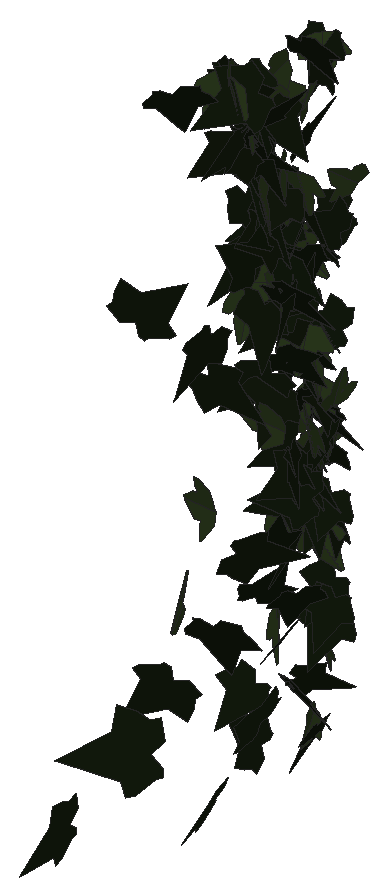
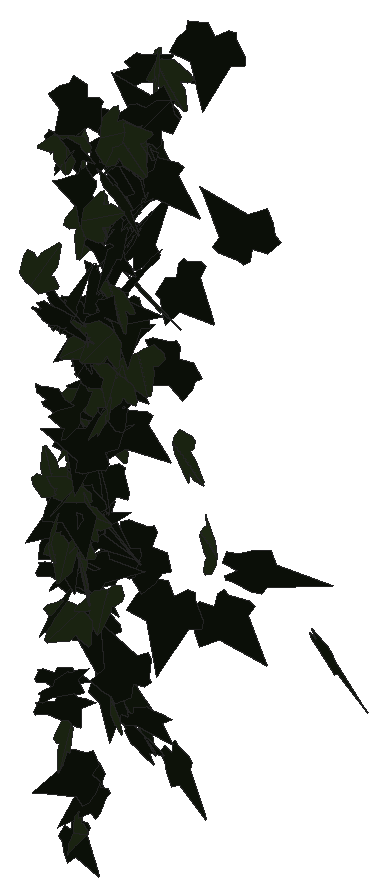
# SketchUp Ruby script. Lengths in inches.
U = 1.inch
M = Sketchup.active_model
def pt(a) = Geom::Point3d.new(a.map { |v| v * U })
def face(e, loops, mat)
  f = e.add_face(loops[0].map { |a| pt(a) })
  loops[1..].each { |l| e.add_face(l.map { |a| pt(a) }).erase! }
  f.material = f.back_material = mat if mat
  f
end
# faces: each face lists its corners as indices into pts; further lists are holes
def faces(e, pts, list, mat = nil) = list.each { |f| face(e, (f[0].is_a?(Array) ? f : [f]).map { |l| l.map { |i| pts[i] } }, mat) }
# xy, xz, yz: faces in a plane at the given z, y or x. An outline is a flat list of corners, or four numbers for a rectangle; further outlines are holes
def ring(l) = l.size == 4 ? [[l[0], l[1]], [l[2], l[1]], [l[2], l[3]], [l[0], l[3]]] : l.each_slice(2).to_a
def flat(e, list, mat, &to3) = list.each { |f| face(e, (f[0].is_a?(Array) ? f : [f]).map { |l| ring(l).map { |u, v| to3.(u, v) } }, mat) }
def xy(e, z, list, mat = nil) = flat(e, list, mat) { |x, y| [x, y, z] }
def xz(e, y, list, mat = nil) = flat(e, list, mat) { |x, z| [x, y, z] }
def yz(e, x, list, mat = nil) = flat(e, list, mat) { |y, z| [x, y, z] }
def lines(e, pts, list) = list.each { |a, b| e.add_line(pt(pts[a]), pt(pts[b])) }
# prism: a flat outline (further loops are holes) pulled along v
def prism(e, loops, v, mat = nil)
  f = face(e, loops, mat); d = Geom::Vector3d.new(v.map { |x| x * U })
  f.pushpull(f.normal.samedirection?(d) ? d.length : -d.length)
end
def box(e, o, s, mat = nil) = prism(e, [[o, [o[0] + s[0], o[1], o[2]], [o[0] + s[0], o[1] + s[1], o[2]], [o[0], o[1] + s[1], o[2]]]], [0, 0, s[2]], mat)
def at(x, y, z, deg = 0) = Geom::Transformation.translation(pt([x, y, z])) * Geom::Transformation.rotation(ORIGIN, Z_AXIS, deg.degrees)
def axes(o, x, y, z) = Geom::Transformation.new([*x, 0, *y, 0, *z, 0, *pt(o).to_a, 1])
def part(name) = M.definitions.add(name)
# library, detail: a bought-in or finely detailed component or shape, given as its bounding box
def library(name, o, s) = part(name).tap { |d| box(d.entities, o, s) }
def detail(e, o, s) = box(e.add_group.entities, o, s)
def put(e, d, t, mat = nil) = e.add_instance(d, t).tap { |i| i.material = mat if mat }
def group(e, t, mat = nil) = e.add_group.tap { |g| g.transformation = t; g.material = mat if mat }.entities
root = M.entities
M.materials.add("efeu1").color = [18, 25, 13]
M.materials.add("efeu2").color = [43, 57, 29]
c1 = part("ivyleaf_9")
p = [[1.54,2.16,1.25],[1.36,2.04,1.19],[-0.21,0.99,0.68],[-0.71,1.11,0.82],[-0.85,0.86,0.67],[-0.8,0.17,0.21],
  [-0.9,-0.01,0.1],[-0.67,-0.16,-0.02],[-0.08,-0.08,-0.05],[-0.03,-0.6,-0.4],[0.65,-0.88,-0.66],[0.83,-0.6,-0.49],
  [1.29,-0.42,-0.43],[1.8125,-0.07,-0.26],[1.21,0.44,0.15]]
faces(c1.entities,p,[[0,1,2,3,4,5,6,7,8,9,10,11,12,13,14]],"efeu1")
c2 = part("ivyleaf_10")
p = [[0,0.5,-0.03],[-0.0625,2.02,-0.43],[-0.19,2.01,-0.46],[-0.54,1.05,-0.29],[-0.52,0.625,-0.18],[-0.83,0.76,-0.28],
  [-1.16,0.64,-0.33],[-1.15,0.33,-0.24],[-0.77,-0.39,0.02],[-0.3,-0.51,0.16],[0.04,-0.48,0.23],[-0.02,2.01,-0.4375],
  [-0.06,2.01,-0.43],[0.04,-0.49,0.23],[0.67,-0.49,0.14],[1.38,0.36,-0.2],[1.375,0.51,-0.24],[0.81,0.65,-0.19],
  [0.62,0.59,-0.15],[0.6,1.09,-0.28],[0.5,1.23,-0.31]]
faces(c2.entities,p,[[0,1,2,3,4,5,6,7,8,9,10],[11,12,0,13,14,15,16,17,18,19,20]],"efeu2")
put(root,c1,axes([503.91,113.92,209.23],[-1.13044,0.58675,-0.20247],[0.17852,-0.10326,-1.2479],[-0.64335,-1.05964,0.00949]))
put(root,c1,axes([506.68,116.01,212.9],[-1.02808,-0.07846,0.94416],[-0.95909,-0.21439,-0.98768],[0.22058,-1.29784,0.10607]))
put(root,c1,axes([503.36,119.53,232.06],[-0.29081,-0.03863,1.11717],[1.11527,-0.31666,0.25736],[0.32221,1.0612,0.11746]))
put(root,c1,axes([504.42,120.57,213.75],[0.18012,0.27174,-1.08192],[-0.63973,-0.85537,-0.33113],[-0.96913,0.61515,0.0175]))
put(root,c2,axes([504.51,120.84,216.73],[0.55223,-0.68279,0.67074],[-0.42151,0.51346,0.88714],[-0.92264,-0.64324,-0.00383]))
put(root,c1,axes([504.11,121.15,242.92],[0.61298,0.85365,-0.28895],[-0.17696,-0.22467,-1.06605],[-0.95325,0.59064,0.0121]))
put(root,c1,axes([505.38,122.09,230.72],[-0.21356,0.4814,-0.97372],[0.43695,-0.84474,-0.54058],[-1.04969,-0.44958,-0.02692]))
put(root,c2,axes([505.26,122.03,222.15],[0.25366,-0.23089,-1.05703],[-0.83814,0.65674,-0.34167],[0.75141,0.81048,-0.02427]))
put(root,c1,axes([505.08,122.75,207.01],[-0.6956,0.73782,-0.30612],[0.20951,-0.22137,-1.01857],[-0.83194,-0.67266,-0.00056]))
put(root,c1,axes([504.72,123.3,215.34],[0.94038,0.5964,-0.48305],[-0.41958,-0.2547,-1.09757],[-0.70033,0.95342,0.00895]))
put(root,c2,axes([504.91,123.83,242.36],[1.06886,0.03727,-0.38639],[-0.40088,-0.0161,-1.03],[-0.0438,1.057,-0.00206]))
put(root,c1,axes([506.02,124.43,242.25],[-0.87747,-0.49721,0.53801],[-0.46341,-0.28969,-0.99041],[0.62109,-0.91859,0.02113]))
put(root,c1,axes([504.26,123.57,227.71],[-0.062,-0.04896,-1.05302],[0.74287,0.74306,-0.07793],[0.80419,-0.69018,-0.0092]))
put(root,c1,axes([505.62,124.84,233.18],[0.12249,0.14041,1.08013],[-0.69224,-0.81721,0.1877],[0.89552,-0.65091,-0.00265]))
put(root,c2,axes([505.15,123.89,242.71],[-0.6354,0.71464,0.49728],[-0.45319,0.26707,-0.95208],[-0.81055,-0.70954,0.14249]))
put(root,c1,axes([505.03,124.7,239.49],[-0.88492,0.69568,-0.18354],[0.14532,-0.1142,-1.11786],[-0.76139,-0.83035,-0.00003]))
put(root,c1,axes([506.34,124.37,210.68],[-0.50135,0.98127,0.40108],[-0.2593,0.31192,-1.12597],[-1.10876,-0.51664,0.08197]))
put(root,c1,axes([505.8,125.07,209.13],[-0.68013,-0.02252,-0.79048],[-0.81959,-0.04413,0.65526],[-0.05221,0.98608,0.01127]))
put(root,c1,axes([504.05,125.69,238.25],[0.09411,0.16165,-0.98413],[-0.58334,-0.77726,-0.18982],[-0.85712,0.54673,0.02113]))
put(root,c1,axes([505.33,126.2,234.09],[0.42909,-0.62707,-0.63231],[0.349,-0.51501,0.77203],[-0.87637,-0.51212,-0.00215]))
put(root,c1,axes([504.9,124.76,218.51],[0.05119,0.4512,-1.02532],[0.17057,0.97343,0.47122],[1.15848,-0.16326,-0.02407]))
put(root,c1,axes([503.53,125.8,240.73],[0.08815,-0.03653,1.11858],[0.90208,-0.678,-0.08987],[0.73288,0.83893,-0.02393]))
put(root,c2,axes([505.71,125.42,236.53],[-0.61081,0.78737,0.2722],[-0.23104,0.16767,-1.00533],[-0.86582,-0.60021,0.07623]))
put(root,c2,axes([504.0625,126.26,239.79],[-0.44832,0.35428,-0.83168],[0.46364,-0.6887,-0.54907],[-0.82302,-0.58096,0.14372]))
put(root,c1,axes([504.38,126.1,238.27],[0.54459,-0.37769,0.82244],[0.74425,-0.39278,-0.65208],[0.58474,0.85168,0.064]))
put(root,c1,axes([504.32,126.42,211.03],[-0.8516,-0.38856,0.02041],[-0.01819,-0.01021,-0.91422],[0.41979,-0.78869,0.00178]))
put(root,c1,axes([504.37,126.4,232.79],[-1.08337,0.15581,-0.30104],[0.27462,-0.22133,-1.04035],[-0.22501,-1.02032,0.1797]))
put(root,c1,axes([503.86,126.29,241.74],[-0.22606,-0.88727,-0.49901],[0.19431,0.44934,-0.94577],[1.07192,-0.26857,0.06621]))
put(root,c2,axes([505.79,126.1,224.6],[-0.10168,0.06196,-0.95999],[-0.97947,0.17709,0.10856],[0.19736,0.9108,0.0442]))
put(root,c1,axes([504.57,126.44,238.3],[-0.11131,-0.09148,-1.05015],[1.07781,0.17004,-0.12195],[0.19332,-1.00067,0.07528]))
put(root,c1,axes([505.27,126.43,218],[0.54921,0.61404,0.50618],[-0.33715,-0.37341,0.82916],[0.77615,-0.5967,0.00201]))
put(root,c1,axes([505.02,125.91,239.54],[0.31741,0.94217,-0.14821],[0.0194,0.14363,1.02608],[1.02894,-0.29335,0.02638]))
put(root,c1,axes([504.51,127,229.83],[0.03094,-1.02309,0.17164],[-0.02579,-0.16571,-1.06403],[1.11892,0.02447,-0.02927]))
put(root,c1,axes([504.49,127.13,239.69],[0.12645,-0.77692,0.53602],[0.14304,-0.50033,-0.81565],[0.99671,0.17037,0.04905]))
put(root,c1,axes([504.12,127.4,236.5],[0.06561,-0.98315,0.16665],[0.01356,-0.16611,-0.98533],[0.99708,0.06695,0.00243]))
put(root,c1,axes([505.29,127.56,235.76],[-0.48589,-0.79099,0.30931],[-0.12041,-0.27843,-0.94553],[0.90468,-0.46188,0.04028]))
put(root,c1,axes([504.75,127.66,225.36],[-0.33744,-0.90752,0.30844],[0.04711,-0.32529,-0.98743],[1.03006,-0.28242,0.1462]))
put(root,c1,axes([504.46,126.92,234.74],[0.57525,-0.69282,-0.45977],[-0.30137,0.34307,-0.90879],[0.83487,0.60121,-0.01125]))
put(root,c1,axes([505.12,126.8,240.01],[0.13198,-0.59195,-0.76682],[-0.05179,0.73862,-0.62497],[1.01987,0.11411,0.06749]))
put(root,c1,axes([504.39,127.47,226.15],[0.07198,0.13744,-0.98481],[-0.32119,-0.89924,-0.15751],[-0.98223,0.30412,-0.02067]))
put(root,c1,axes([505.6875,127.43,230.98],[-0.63476,0.20011,-0.74659],[0.73131,-0.23844,-0.64568],[-0.33615,-0.89662,0.00508]))
put(root,c2,axes([504.38,127.47,240.55],[-0.66308,-0.50809,0.5812],[-0.39207,-0.43304,-0.82424],[0.71532,-0.70834,0.08699]))
put(root,c2,axes([503.27,127.51,229.81],[0.53452,0.89946,-0.25334],[-0.19046,-0.18043,-1.06552],[-0.98823,0.52128,0.06833]))
put(root,c1,axes([505.28,127.02,230.9375],[1.11683,0.14517,0.15296],[0.15011,0.06678,-1.08494],[-0.16515,1.04237,0.04821]))
put(root,c1,axes([502.99,127.63,234.55],[0.37351,-0.88306,-0.24384],[-0.06487,0.23718,-0.95828],[0.9138,0.37778,0.03164]))
put(root,c1,axes([505.24,127.98,222.25],[-0.17927,-0.17288,-0.8841],[0.9341,-0.09986,-0.15452],[-0.0724,-0.86038,0.19558]))
put(root,c1,axes([506.04,127.37,215.73],[0.18545,0.82023,-0.35116],[-0.11185,-0.32303,-0.87087],[-0.95142,0.19785,0.03394]))
put(root,c1,axes([503.56,127.31,237.06],[0.79779,-0.49957,-0.60287],[-0.40582,0.46509,-0.91482],[0.71997,0.81571,0.15238]))
put(root,c1,axes([504.97,128.04,229.21],[0.04356,0.22846,-0.94856],[-0.21862,-0.8894,-0.24101],[-0.99166,0.20611,0.01146]))
put(root,c2,axes([505.19,127.48,236.83],[-0.59647,0.78335,0.28517],[-0.45403,0.01994,-0.93987],[-0.77285,-0.61628,0.33206]))
put(root,c1,axes([505.25,128.46,221.03],[-0.33617,-0.49235,0.67588],[-0.35401,-0.56137,-0.60559],[0.80626,-0.45178,0.01591]))
put(root,c2,axes([504.37,128.46,241.24],[0.00909,0.30255,-1.01224],[-0.275,-0.94186,-0.30677],[-1.06589,0.24558,0.07052]))
put(root,c1,axes([505.49,128.09,218.13],[-0.65372,0.26218,-0.58366],[0.48535,-0.35416,-0.67615],[-0.46041,-0.74559,0.11593]))
put(root,c1,axes([506.24,128,220.4],[-0.8371,0.20759,0.60284],[-0.61284,0.12083,-0.83413],[-0.25807,-0.9603,0.02536]))
put(root,c1,axes([504.6,127.63,238.11],[-0.4298,0.71274,0.457],[-0.30666,0.34282,-0.84574],[-0.85071,-0.48367,0.07398]))
put(root,c2,axes([504.82,127.8,230.22],[0.57365,-0.31226,-0.75791],[-0.61319,0.46245,-0.63645],[0.59766,0.77418,0.07448]))
put(root,c1,axes([504.92,127.56,227.27],[0.93791,0.51564,0.14264],[0.14068,0.04917,-1.05008],[-0.55882,0.87782,-0.02496]))
put(root,c2,axes([505.75,128.03,236.28],[-0.97486,0.08176,-0.02505],[0.02573,-0.00393,-0.9426],[-0.08838,-0.90296,0.00183]))
put(root,c1,axes([505.55,127.38,232.35],[0.04571,0.40058,0.96168],[0.04502,0.92402,-0.41828],[-1.08741,0.05509,0.0231]))
put(root,c1,axes([503.8125,127.79,232.6],[-0.05505,0.98433,0.10408],[-0.02334,0.09908,-1.02494],[-1.06831,-0.05289,0.01703]))
put(root,c1,axes([504.7,127.76,212.65],[-0.10379,0.8023,0.30586],[-0.03092,0.29276,-0.84034],[-0.92235,-0.1001,-0.00625]))
put(root,c1,axes([504.72,128.09,231.92],[0.59958,-0.60968,-0.48435],[-0.14197,0.51547,-0.82459],[0.76561,0.57305,0.22641]))
put(root,c1,axes([505.27,128.27,229.15],[-0.95994,-0.37987,0.10233],[0.10434,0.02427,1.00514],[-0.41075,0.89393,0.01619]))
put(root,c1,axes([504.19,128.72,235.66],[-0.77554,-0.22596,-0.57955],[0.56212,0.20113,-0.78235],[0.32524,-0.88642,-0.02978]))
put(root,c2,axes([506.05,127.97,240.08],[0.38293,-0.1606,0.85179],[-0.56184,0.65334,0.36745],[-0.70488,-0.608,0.16986]))
put(root,c1,axes([502.9375,128.51,214.1],[0.74859,0.63391,0.141],[-0.10958,-0.08995,0.97687],[0.69148,-0.70052,0.00215]))
put(root,c1,axes([504.83,129.2,219.35],[-0.14693,-0.34635,-0.80924],[-0.14613,-0.76918,0.38067],[-0.90817,0.1798,0.06967]))
put(root,c1,axes([505.17,128.57,221.75],[0.78581,-0.62595,-0.20129],[-0.04214,0.24732,-0.98443],[0.70635,0.71112,0.1652]))
put(root,c2,axes([505.97,128.43,223.89],[-0.86075,0.53702,0.30259],[-0.29508,0.11431,-0.99781],[-0.58995,-0.8407,0.05761]))
put(root,c2,axes([503.48,129.05,212.9],[0.59692,-0.44382,0.6469],[0.58976,-0.30758,-0.73286],[0.57726,0.77317,0.0798]))
put(root,c1,axes([503.79,129.44,232.9],[-0.04021,-0.34128,-0.91152],[-0.1401,-0.8669,0.35679],[-1.0061,0.13436,-0.01325]))
put(root,c1,axes([504.46,128.79,222.14],[-0.84006,0.48385,0.12629],[-0.12223,0.04792,-0.95248],[-0.52472,-0.78579,0.01968]))
put(root,c2,axes([505.28,128.89,227.89],[0.8614,0.44883,-0.10175],[-0.10187,-0.03184,-0.95162],[-0.48555,0.80294,0.01914]))
put(root,c1,axes([505.39,128.32,237.76],[-0.18095,0.83482,-0.34618],[-0.25602,0.28556,0.86892],[0.93626,0.23943,0.1707]))
put(root,c1,axes([505.41,128.65,242.71],[0.96701,0.25916,-0.16492],[-0.16183,-0.05263,-0.96937],[-0.28545,0.90779,-0.00912]))
put(root,c1,axes([504.43,128.39,224.26],[0.28151,0.97299,0.20348],[0.05205,0.18964,-1.04759],[-1.0706,0.26507,0.00257]))
put(root,c2,axes([503.36,129.19,233.92],[0.98247,-0.3343,-0.05841],[-0.05397,0.02684,-1.00791],[0.3621,0.91103,0.00826]))
put(root,c1,axes([503.28,128.84,236.75],[0.79184,-0.22157,-0.6024],[-0.58795,0.19965,-0.79608],[0.3208,0.9128,0.0279]))
put(root,c1,axes([504.04,129.33,226.81],[0.66372,-0.68917,-0.03715],[-0.03815,0.01483,-0.95665],[0.68911,0.66459,-0.01718]))
put(root,c1,axes([505.28,129.58,219.36],[0.00661,-0.89381,-0.10106],[-0.00099,0.09717,-0.92958],[0.971,0.00618,-0.00026]))
put(root,c1,axes([505.11,128.91,231.98],[0.52865,0.71027,-0.23967],[-0.15347,-0.18191,-0.89701],[-0.79172,0.50953,0.01385]))
put(root,c1,axes([506.33,129.15,222.71],[-0.67978,0.655,0.00955],[-0.00752,0.00605,-0.94474],[-0.70743,-0.62946,0.00087]))
put(root,c2,axes([503.81,129.21,218.4],[0.32435,0.94552,0.08475],[0.0247,0.07824,-1.03175],[-1.02465,0.30119,0.00195]))
put(root,c1,axes([505.87,129.91,219.57],[-0.72752,-0.65486,-0.09962],[0.09423,0.04761,-0.97667],[0.70854,-0.67874,0.0276]))
put(root,c2,axes([502.87,129.56,229.82],[0.95049,-0.01983,0.41316],[0.42957,0.05154,-0.91372],[-0.00341,0.96422,0.05734]))
put(root,c2,axes([505.64,129.15,222.54],[-0.72117,0.55308,0.53297],[-0.43162,0.32086,-0.90171],[-0.69052,-0.77818,0.007]))
put(root,c1,axes([505.54,130.11,232.14],[0.48227,-0.84067,0.17557],[-0.07007,0.15666,0.98985],[-0.9234,-0.45095,0.01658]))
put(root,c1,axes([504.41,129.92,221.26],[0.27265,-0.86727,-0.22469],[-0.02232,0.22822,-0.90796],[0.89562,0.26971,0.04577]))
put(root,c1,axes([505.875,130.15,214.18],[-0.66254,-0.52603,-0.17107],[0.14987,0.09077,-0.84015],[0.57606,-0.62862,0.02184]))
put(root,c2,axes([503.25,129.97,228.16],[-0.10347,0.80869,-0.37147],[0.05517,-0.35361,-0.84687],[-0.95318,-0.10825,-0.00869]))
put(root,c2,axes([505.125,129.89,226.33],[-0.18594,0.81163,-0.25397],[0.03,-0.24365,-0.86256],[-0.91489,-0.17294,0.02333]))
put(root,c1,axes([505.04,130.53,240.6875],[-0.1734,-0.42586,0.80442],[0.06762,-0.78967,-0.43866],[0.9512,-0.02149,0.17782]))
put(root,c1,axes([504.91,129.42,230.54],[0.21814,-0.10473,0.89187],[-0.24143,0.84436,0.162],[-0.90128,-0.25154,0.17247]))
put(root,c1,axes([503,130.18,223.85],[-0.08751,0.34413,0.83045],[0.1767,-0.7816,0.36759],[0.92229,0.1824,0.00837]))
put(root,c2,axes([503.45,130.64,238.21],[0.0289,-0.11863,0.94329],[0.04068,-0.90649,-0.12446],[0.98708,0.04083,-0.02249]))
put(root,c2,axes([503.93,129.79,231.5],[0.52121,0.20819,0.79691],[0.71363,0.39195,-0.54356],[-0.47555,0.81635,0.05774]))
put(root,c2,axes([504.94,130.05,217.36],[-0.81914,-0.1766,-0.59573],[0.64137,-0.0959,-0.78704],[0.08793,-0.94561,0.19107]))
put(root,c1,axes([504.49,129.79,226.51],[0.72359,0.35843,-0.44802],[-0.43056,-0.16704,-0.78937],[-0.42536,0.77882,0.03689]))
put(root,c1,axes([506.2,130.2,227.93],[-0.60918,0.20872,0.63911],[-0.63439,0.18208,-0.62503],[-0.29809,-0.81404,0.02407]))
put(root,c1,axes([506.35,129.92,233],[-0.45483,0.40561,0.659],[-0.50496,0.42782,-0.60799],[-0.63659,-0.62916,0.01142]))
put(root,c1,axes([505.42,130.7,213.1],[-0.65176,-0.6984,-0.03704],[0.05599,0.00224,-0.95913],[0.75317,-0.60452,0.03924]))
put(root,c1,axes([503.54,130.05,209.18],[0.95999,-0.19867,-0.09245],[-0.08767,0.04419,-0.94688],[0.2181,0.89222,0.02631]))
put(root,c2,axes([502.99,130.2,232.19],[-0.80986,0.06113,-0.51857],[0.53318,-0.07609,-0.78184],[-0.10038,-0.8973,0.03097]))
put(root,c1,axes([504.64,130.73,223.97],[0.29606,-0.82749,0.20964],[0.09837,-0.18206,-0.9061],[0.91455,0.28746,0.0296]))
put(root,c2,axes([504.12,130.15,222.8],[0.29029,0.01719,0.89216],[-0.92072,0.10699,0.27557],[-0.10478,-0.89258,0.05022]))
put(root,c1,axes([504.1,130.74,228.23],[0.5797,-0.61483,0.35786],[0.23214,-0.26905,-0.84869],[0.72465,0.57803,-0.0144]))
put(root,c2,axes([505.66,130.65,224.02],[-0.08656,-0.84707,-0.05641],[0.03596,-0.05757,0.88398],[-0.916,0.07779,0.04003]))
put(root,c1,axes([503.16,130.24,226.43],[0.34264,-0.07296,0.90207],[0.93588,0.11365,-0.31969],[-0.08877,0.91656,0.11145]))
put(root,c1,axes([504.4375,130.73,206.96],[-0.42382,0.52832,-0.52313],[0.29719,-0.42177,-0.68397],[-0.72963,-0.47868,0.02528]))
put(root,c1,axes([505.12,131.14,217.77],[0.15217,-0.71636,0.51232],[0.10782,-0.48241,-0.75927],[0.93273,0.17263,0.00419]))
put(root,c1,axes([504.04,130.08,209.64],[0.64776,0.27679,0.55714],[0.53897,0.19626,-0.68653],[-0.36554,0.77987,-0.02497]))
put(root,c1,axes([504.8125,130.9,241.82],[-0.75713,-0.29931,-0.4442],[0.45745,0.09079,-0.78919],[0.32867,-0.81587,0.07514]))
put(root,c2,axes([504.52,130.54,224.13],[0.72979,0.30837,0.47191],[0.45148,0.17679,-0.7724],[-0.38371,0.79451,-0.01129]))
put(root,c1,axes([504.62,130.28,223.59],[0.38499,0.70902,-0.53504],[-0.61954,-0.23084,-0.74423],[-0.71501,0.58177,0.35677]))
put(root,c2,axes([504.8125,130.64,241.65],[0.71854,0.56447,0.04609],[0.03613,0.02907,-0.90741],[-0.61044,0.66615,0.00054]))
put(root,c2,axes([503.99,131.15,207.25],[-0.04702,0.43113,-0.7345],[0.01421,-0.70678,-0.44955],[-0.89353,-0.03393,0.03151]))
put(root,c1,axes([504.95,131.3,214.39],[-0.37476,-0.74451,0.31525],[-0.15106,-0.2692,-0.85417],[0.85492,-0.37393,-0.01274]))
put(root,c1,axes([505.11,130.59,221.58],[0.41418,0.39412,-0.66104],[-0.64095,-0.2743,-0.54929],[-0.49152,0.6898,0.15926]))
put(root,c2,axes([505.99,131.4,234.76],[-0.40961,-0.40888,-0.70981],[-0.31326,-0.63299,0.56201],[-0.80012,0.45715,0.14333]))
put(root,c2,axes([503.77,130.91,220.74],[0.56361,-0.73561,-0.07785],[-0.01494,0.08653,-0.92582],[0.73957,0.56235,0.04062]))
put(root,c1,axes([504.625,130.65,223.03],[0.91975,-0.06002,0.11284],[0.11703,-0.0057,-0.88788],[0.06508,0.85848,0.00199]))
put(root,c2,axes([504.85,130.67,211.75],[-0.73367,0.52352,0.1528],[-0.12024,0.09622,-0.89191],[-0.5748,-0.68833,-0.00846]))
put(root,c1,axes([505.6,131.21,233.09],[-0.96156,0.02482,0.23529],[-0.2446,-0.00614,-0.92622],[-0.02434,-0.9186,0.01255]))
put(root,c2,axes([504.85,131.61,221.77],[0.08874,-0.15545,0.88059],[0.55921,-0.67059,-0.1803],[0.74277,0.52344,0.03053]))
put(root,c2,axes([504.47,130.95,221.68],[-0.5817,-0.67162,-0.25607],[0.16245,0.19498,-0.89534],[0.75529,-0.5592,-0.00464]))
